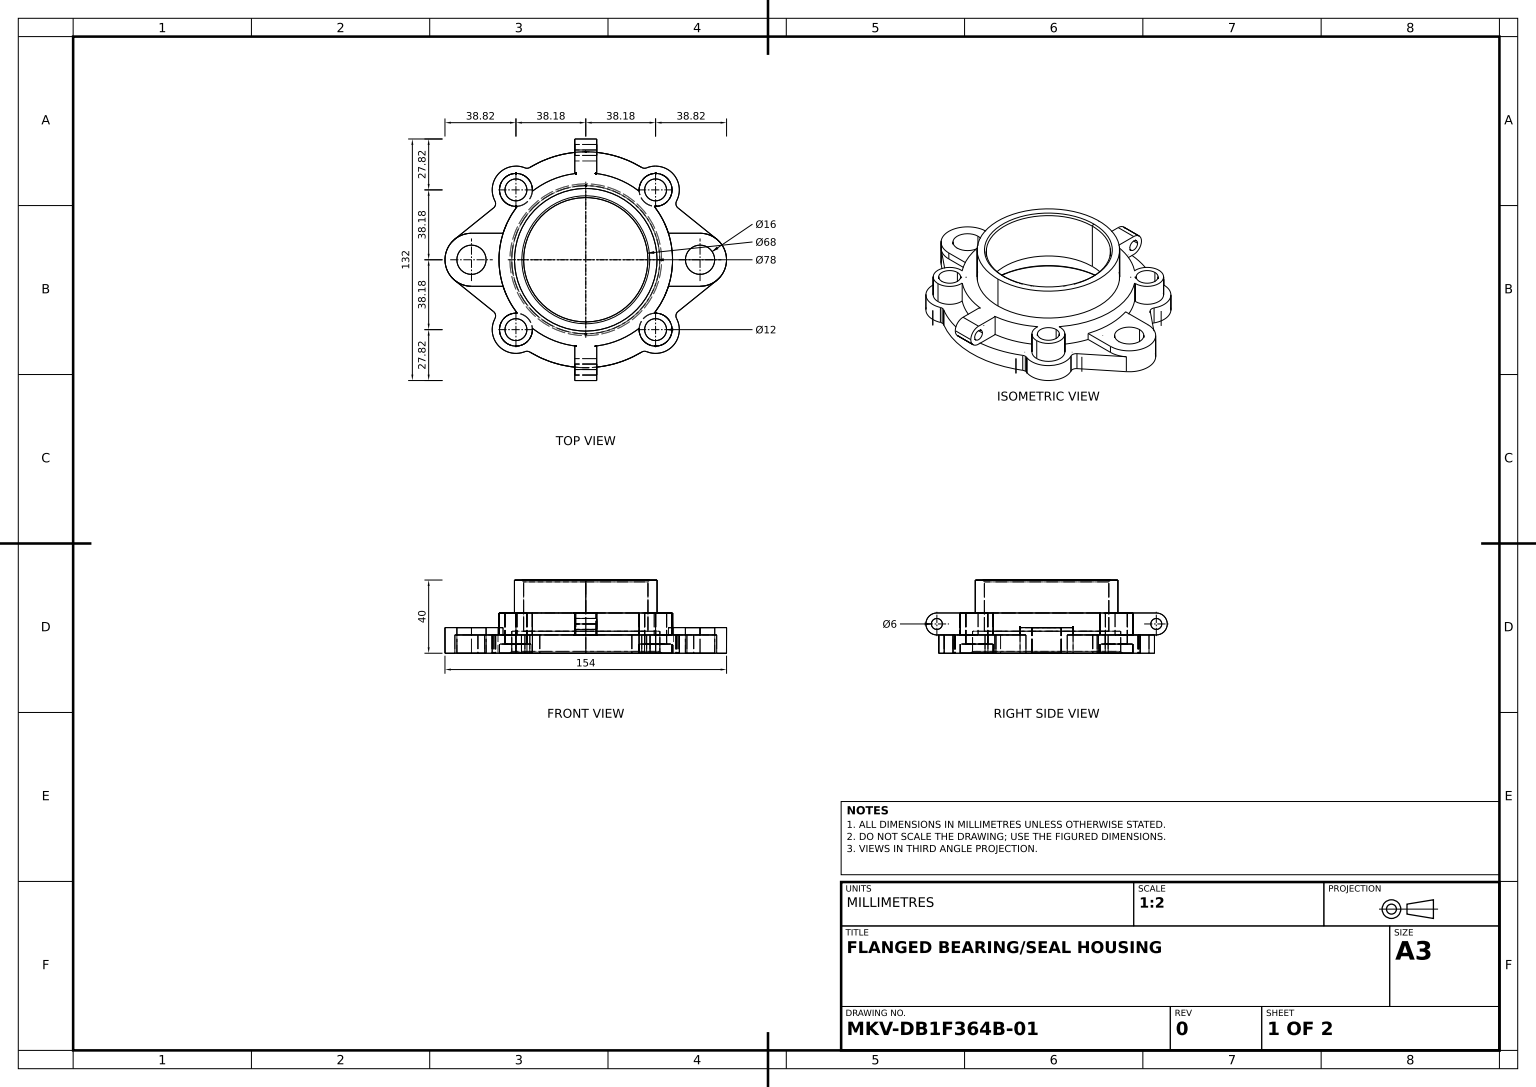
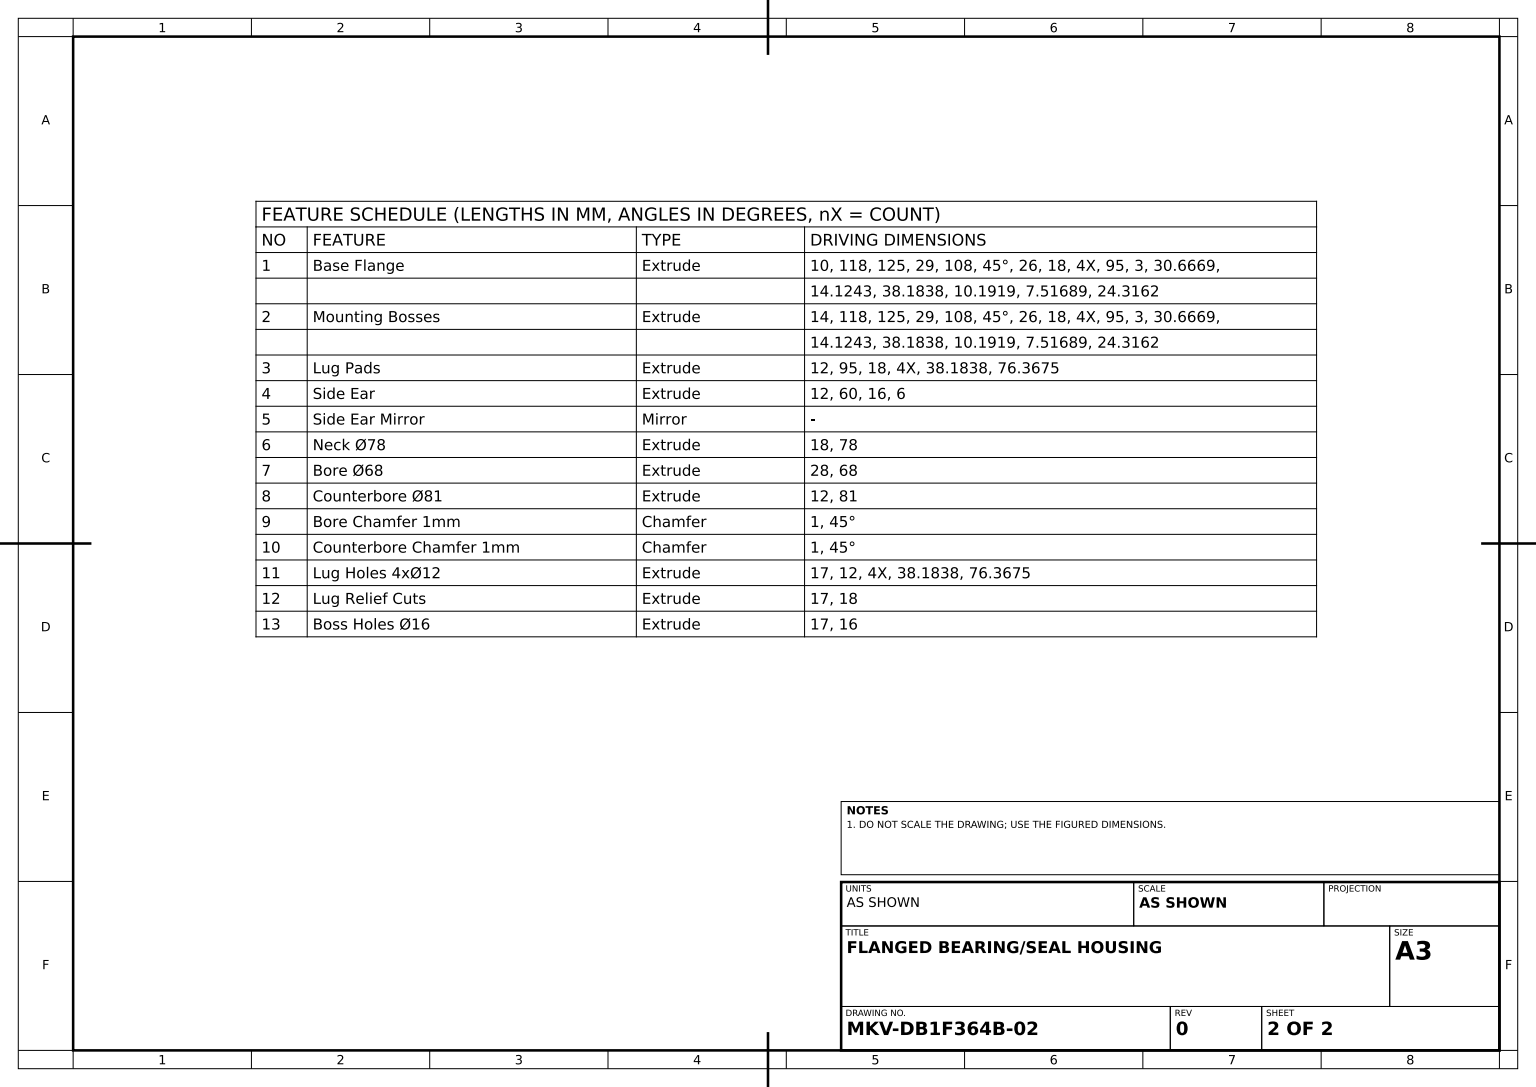
solid
v1 (38.183766,5,-32.183766)
v2 (38.183766,22,-32.183766)
e1 v1 v2 LINE
v3 (38.183766,22,-44.183766)
e2 v2 v3 CIRCLE(AX(P(38.183766,22,-38.183766),D(0,1,0),D(0,0,1)),6)
v4 (38.183766,5,-44.183766)
e3 v4 v3 LINE
e4 v1 v4 CIRCLE(AX(P(38.183766,5,-38.183766),D(0,1,0),D(0,0,1)),6)
face CYL(AX(P(38.183766,5,-38.183766),D(0,1,0),D(0,0,1)),6) rev [e1 e2 -e3 -e4]
v5 (6,16,-63)
v6 (-6,16,-63)
e5 v5 v6 LINE
v7 (6,16,-57)
e6 v7 v5 CIRCLE(AX(P(6,16,-60),D(-1,0,0),D(0,0,1)),3)
v8 (-6,16,-57)
e7 v7 v8 LINE
e8 v8 v6 CIRCLE(AX(P(-6,16,-60),D(-1,0,0),D(0,0,1)),3)
face CYL(AX(P(6,16,-60),D(-1,0,0),D(0,0,1)),3) rev [-e5 -e6 e7 e8]
v9 (-29.213373,22,37.454357)
v10 (-29.213373,10,37.454357)
e9 v9 v10 LINE
v11 (-38.183766,22,47.183766)
e10 v11 v9 CIRCLE(AX(P(-38.183766,22,38.183766),D(0,1,0),D(0,0,1)),9)
v12 (-38.183766,10,47.183766)
e11 v11 v12 LINE
e12 v12 v10 CIRCLE(AX(P(-38.183766,10,38.183766),D(0,1,0),D(0,0,1)),9)
face CYL(AX(P(-38.183766,22,38.183766),D(0,-1,0),D(0,0,-1)),9) [-e9 -e10 e11 e12]
v13 (-38.183766,0,-29.183766)
v14 (-38.183766,0,-47.183766)
e13 v13 v14 CIRCLE(AX(P(-38.183766,0,-38.183766),D(0,1,0),D(0,0,1)),9)
v15 (-38.183766,5,-29.183766)
e14 v13 v15 LINE
v16 (-38.183766,5,-47.183766)
e15 v15 v16 CIRCLE(AX(P(-38.183766,5,-38.183766),D(0,1,0),D(0,0,1)),9)
e16 v14 v16 LINE
face CYL(AX(P(-38.183766,-12,-38.183766),D(0,1,0),D(0,0,1)),9) rev [-e13 e14 e15 -e16]
v17 (38.183766,0,47.183766)
v18 (38.183766,5,47.183766)
e17 v17 v18 LINE
v19 (38.183766,5,29.183766)
e18 v18 v19 CIRCLE(AX(P(38.183766,5,38.183766),D(0,1,0),D(0,0,1)),9)
v20 (38.183766,0,29.183766)
e19 v20 v19 LINE
e20 v17 v20 CIRCLE(AX(P(38.183766,0,38.183766),D(0,1,0),D(0,0,1)),9)
face CYL(AX(P(38.183766,-12,38.183766),D(0,1,0),D(0,0,1)),9) rev [e17 e18 -e19 -e20]
v21 (38.183766,22,-47.183766)
v22 (38.183766,10,-47.183766)
e21 v21 v22 LINE
v23 (29.213373,10,-37.454357)
e22 v22 v23 CIRCLE(AX(P(38.183766,10,-38.183766),D(0,1,0),D(0,0,1)),9)
v24 (29.213373,22,-37.454357)
e23 v24 v23 LINE
e24 v21 v24 CIRCLE(AX(P(38.183766,22,-38.183766),D(0,1,0),D(0,0,1)),9)
face CYL(AX(P(38.183766,22,-38.183766),D(0,-1,0),D(0,0,-1)),9) [e21 e22 -e23 -e24]
v25 (-50.427104,0,-28.329799)
v26 (-71.591397,0,-11.295862)
e25 v25 v26 LINE
v27 (-71.591397,10,-11.295862)
e26 v27 v26 LINE
v28 (-50.427104,10,-28.329799)
e27 v28 v27 LINE
e28 v28 v25 LINE
face PLANE(AX(P(-33.661405,10,-41.823557),D(0.626992924,0,0.77902495),D(0.77902495,0,-0.626992924))) rev [e25 -e26 -e27 e28]
e29 v3 v2 CIRCLE(AX(P(38.183766,22,-38.183766),D(0,1,0),D(0,0,1)),6)
e30 v4 v1 CIRCLE(AX(P(38.183766,5,-38.183766),D(0,1,0),D(0,0,1)),6)
face CYL(AX(P(38.183766,5,-38.183766),D(0,1,0),D(0,0,1)),6) rev [e3 e29 -e1 -e30]
v29 (0,39,-34)
v30 (0,40,-35)
e31 v29 v30 LINE
v31 (0,39,34)
e32 v31 v29 CIRCLE(AX(P(0,39,0),D(0,1,0),D(0,0,1)),34)
v32 (0,40,35)
e33 v31 v32 LINE
e34 v30 v32 CIRCLE(AX(P(0,40,0),D(0,-1,0),D(0,0,1)),35)
face CONE(AX(P(0,39,0),D(0,1,0),D(0,0,1)),34,0.785398163) rev [-e31 -e32 e33 -e34]
v33 (62.5,0,-8)
v34 (62.5,14,-8)
e35 v33 v34 LINE
v35 (62.5,14,8)
e36 v34 v35 CIRCLE(AX(P(62.5,14,0),D(0,1,0),D(0,0,1)),8)
v36 (62.5,0,8)
e37 v36 v35 LINE
e38 v33 v36 CIRCLE(AX(P(62.5,0,0),D(0,1,0),D(0,0,1)),8)
face CYL(AX(P(62.5,-3,0),D(0,1,0),D(0,0,1)),8) rev [e35 e36 -e37 -e38]
v37 (0,10,-59)
v38 (0,0,-59)
e39 v37 v38 LINE
v39 (6,10,-58.694122)
e40 v37 v39 CIRCLE(AX(P(0,10,0),D(0,-1,0),D(0,0,-1)),59)
v40 (30.604247,10,-50.441848)
e41 v40 v39 CIRCLE(AX(P(0,10,0),D(0,1,0),D(0,0,1)),59)
v41 (30.604247,0,-50.441848)
e42 v40 v41 LINE
e43 v41 v38 CIRCLE(AX(P(0,0,0),D(0,1,0),D(0,0,1)),59)
face CYL(AX(P(0,10,0),D(0,-1,0),D(0,0,-1)),59) [-e39 e40 -e41 e42 e43]
v42 (29.213373,22,37.454357)
v43 (29.213373,10,37.454357)
e44 v42 v43 LINE
v44 (38.183766,10,47.183766)
e45 v43 v44 CIRCLE(AX(P(38.183766,10,38.183766),D(0,1,0),D(0,0,1)),9)
v45 (38.183766,22,47.183766)
e46 v45 v44 LINE
e47 v42 v45 CIRCLE(AX(P(38.183766,22,38.183766),D(0,1,0),D(0,0,1)),9)
face CYL(AX(P(38.183766,22,38.183766),D(0,-1,0),D(0,0,-1)),9) [e44 e45 -e46 -e47]
v46 (-37.454357,22,29.213373)
v47 (-37.454357,10,29.213373)
e48 v46 v47 LINE
v48 (-38.183766,10,29.183766)
e49 v47 v48 CIRCLE(AX(P(-38.183766,10,38.183766),D(0,1,0),D(0,0,1)),9)
v49 (-38.183766,22,29.183766)
e50 v49 v48 LINE
e51 v46 v49 CIRCLE(AX(P(-38.183766,22,38.183766),D(0,1,0),D(0,0,1)),9)
face CYL(AX(P(-38.183766,22,38.183766),D(0,-1,0),D(0,0,-1)),9) [e48 e49 -e50 -e51]
v50 (-38.183766,5,29.183766)
v51 (-38.183766,5,47.183766)
e52 v50 v51 CIRCLE(AX(P(-38.183766,5,38.183766),D(0,1,0),D(0,0,1)),9)
v52 (-38.183766,0,47.183766)
e53 v52 v51 LINE
v53 (-38.183766,0,29.183766)
e54 v53 v52 CIRCLE(AX(P(-38.183766,0,38.183766),D(0,1,0),D(0,0,1)),9)
e55 v53 v50 LINE
face CYL(AX(P(-38.183766,-12,38.183766),D(0,1,0),D(0,0,1)),9) rev [e52 -e53 -e54 e55]
v54 (0,40,39)
v55 (0,40,-39)
e56 v54 v55 CIRCLE(AX(P(0,40,0),D(0,1,0),D(0,0,1)),39)
v56 (0,22,39)
e57 v54 v56 LINE
v57 (0,22,-39)
e58 v56 v57 CIRCLE(AX(P(0,22,0),D(0,1,0),D(0,0,1)),39)
e59 v55 v57 LINE
face CYL(AX(P(0,40,0),D(0,-1,0),D(0,0,-1)),39) [-e56 e57 e58 -e59]
v58 (38.183766,0,-29.183766)
v59 (38.183766,5,-29.183766)
e60 v58 v59 LINE
v60 (38.183766,5,-47.183766)
e61 v59 v60 CIRCLE(AX(P(38.183766,5,-38.183766),D(0,1,0),D(0,0,1)),9)
v61 (38.183766,0,-47.183766)
e62 v61 v60 LINE
e63 v58 v61 CIRCLE(AX(P(38.183766,0,-38.183766),D(0,1,0),D(0,0,1)),9)
face CYL(AX(P(38.183766,-12,-38.183766),D(0,1,0),D(0,0,1)),9) rev [e60 e61 -e62 -e63]
e64 v5 v7 CIRCLE(AX(P(6,16,-60),D(-1,0,0),D(0,0,1)),3)
e65 v6 v8 CIRCLE(AX(P(-6,16,-60),D(-1,0,0),D(0,0,1)),3)
face CYL(AX(P(6,16,-60),D(-1,0,0),D(0,0,1)),3) rev [-e64 e5 e65 -e7]
v62 (38.183766,22,-29.183766)
e66 v62 v21 CIRCLE(AX(P(38.183766,22,-38.183766),D(0,1,0),D(0,0,1)),9)
v63 (38.183766,10,-29.183766)
e67 v62 v63 LINE
e68 v63 v22 CIRCLE(AX(P(38.183766,10,-38.183766),D(0,1,0),D(0,0,1)),9)
face CYL(AX(P(38.183766,22,-38.183766),D(0,-1,0),D(0,0,-1)),9) [-e66 e67 e68 -e21]
v64 (38.183766,5,44.183766)
v65 (38.183766,5,32.183766)
e69 v64 v65 CIRCLE(AX(P(38.183766,5,38.183766),D(0,1,0),D(0,0,1)),6)
v66 (38.183766,22,44.183766)
e70 v64 v66 LINE
v67 (38.183766,22,32.183766)
e71 v66 v67 CIRCLE(AX(P(38.183766,22,38.183766),D(0,1,0),D(0,0,1)),6)
e72 v65 v67 LINE
face CYL(AX(P(38.183766,5,38.183766),D(0,1,0),D(0,0,1)),6) rev [-e69 e70 e71 -e72]
v68 (-38.183766,5,44.183766)
v69 (-38.183766,5,32.183766)
e73 v68 v69 CIRCLE(AX(P(-38.183766,5,38.183766),D(0,1,0),D(0,0,1)),6)
e74 v69 v68 CIRCLE(AX(P(-38.183766,5,38.183766),D(0,1,0),D(0,0,1)),6)
e75 v51 v50 CIRCLE(AX(P(-38.183766,5,38.183766),D(0,1,0),D(0,0,1)),9)
face PLANE(AX(P(-38.183766,5,38.183766),D(0,1,0),D(0,0,1))) rev [e73 e74] [-e75 -e52]
v70 (-62.5,0,8)
v71 (-62.5,0,-8)
e76 v70 v71 CIRCLE(AX(P(-62.5,0,0),D(0,1,0),D(0,0,1)),8)
v72 (-62.5,14,8)
e77 v70 v72 LINE
v73 (-62.5,14,-8)
e78 v72 v73 CIRCLE(AX(P(-62.5,14,0),D(0,1,0),D(0,0,1)),8)
e79 v71 v73 LINE
face CYL(AX(P(-62.5,-3,0),D(0,1,0),D(0,0,1)),8) rev [-e76 e77 e78 -e79]
v74 (-62.5,14,-14.5)
v75 (-45.232732,14,-14.5)
e80 v74 v75 LINE
v76 (-45.232732,10,-14.5)
e81 v75 v76 LINE
v77 (-62.5,10,-14.5)
e82 v77 v76 LINE
e83 v74 v77 LINE
face PLANE(AX(P(0,14,-14.5),D(0,0,-1),D(-1,0,0))) [e80 e81 -e82 -e83]
e84 v55 v54 CIRCLE(AX(P(0,40,0),D(0,1,0),D(0,0,1)),39)
e85 v32 v30 CIRCLE(AX(P(0,40,0),D(0,-1,0),D(0,0,1)),35)
face PLANE(AX(P(0,40,0),D(0,1,0),D(0,0,1))) [e84 e56] [e85 e34]
v78 (37.454357,10,-29.213373)
e86 v78 v63 CIRCLE(AX(P(38.183766,10,-38.183766),D(0,1,0),D(0,0,1)),9)
v79 (37.454357,22,-29.213373)
e87 v79 v62 CIRCLE(AX(P(38.183766,22,-38.183766),D(0,1,0),D(0,0,1)),9)
e88 v79 v78 LINE
face CYL(AX(P(38.183766,22,-38.183766),D(0,-1,0),D(0,0,-1)),9) [e86 -e67 -e87 e88]
v80 (-49.659774,10,-32.076291)
e89 v28 v80 CIRCLE(AX(P(-52.308083,10,-30.666874),D(0,1,0),D(0,0,1)),3)
v81 (-49.659774,0,-32.076291)
e90 v80 v81 LINE
e91 v25 v81 CIRCLE(AX(P(-52.308083,0,-30.666874),D(0,1,0),D(0,0,1)),3)
face CYL(AX(P(-52.308083,10,-30.666874),D(0,-1,0),D(0,0,-1)),3) rev [-e28 e89 e90 -e91]
e92 v35 v34 CIRCLE(AX(P(62.5,14,0),D(0,1,0),D(0,0,1)),8)
v82 (62.5,14,14.5)
v83 (62.5,14,-14.5)
e93 v82 v83 CIRCLE(AX(P(62.5,14,0),D(0,1,0),D(0,0,1)),14.5)
v84 (45.232732,14,-14.5)
e94 v83 v84 LINE
v85 (45.232732,14,14.5)
e95 v85 v84 CIRCLE(AX(P(0,14,0),D(0,1,0),D(0,0,1)),47.5)
e96 v82 v85 LINE
face PLANE(AX(P(0,14,0),D(0,1,0),D(0,0,1))) [-e92 -e36] [e93 e94 -e95 -e96]
v86 (0,12,34)
e97 v86 v31 LINE
v87 (0,12,-34)
e98 v87 v29 LINE
e99 v86 v87 CIRCLE(AX(P(0,12,0),D(0,1,0),D(0,0,1)),34)
face CYL(AX(P(0,12,0),D(0,1,0),D(0,0,1)),34) rev [e97 e32 -e98 -e99]
v88 (5.471947,10,47.183766)
v89 (5.471947,22,47.183766)
e100 v88 v89 LINE
e101 v88 v43 CIRCLE(AX(P(0,10,0),D(0,1,0),D(0,0,1)),47.5)
e102 v89 v42 CIRCLE(AX(P(0,22,0),D(0,1,0),D(0,0,1)),47.5)
face CYL(AX(P(0,22,0),D(0,-1,0),D(0,0,-1)),47.5) [-e100 e101 -e44 -e102]
v90 (6,16,57)
v91 (-6,16,57)
e103 v90 v91 LINE
v92 (6,16,63)
e104 v90 v92 CIRCLE(AX(P(6,16,60),D(1,0,0),D(0,0,-1)),3)
v93 (-6,16,63)
e105 v92 v93 LINE
e106 v91 v93 CIRCLE(AX(P(-6,16,60),D(1,0,0),D(0,0,-1)),3)
face CYL(AX(P(6,16,60),D(-1,0,0),D(0,0,1)),3) rev [-e103 e104 e105 -e106]
v94 (-6,10,-58.694122)
e107 v94 v37 CIRCLE(AX(P(0,10,0),D(0,-1,0),D(0,0,-1)),59)
v95 (-30.604247,0,-50.441848)
e108 v38 v95 CIRCLE(AX(P(0,0,0),D(0,1,0),D(0,0,1)),59)
v96 (-30.604247,10,-50.441848)
e109 v96 v95 LINE
e110 v94 v96 CIRCLE(AX(P(0,10,0),D(0,1,0),D(0,0,1)),59)
face CYL(AX(P(0,10,0),D(0,-1,0),D(0,0,-1)),59) [e107 e39 e108 -e109 -e110]
v97 (62.5,10,14.5)
v98 (45.232732,10,14.5)
e111 v97 v98 LINE
e112 v82 v97 LINE
e113 v85 v98 LINE
face PLANE(AX(P(0,14,14.5),D(0,0,1),D(1,0,0))) [-e111 -e112 e96 e113]
e114 v16 v15 CIRCLE(AX(P(-38.183766,5,-38.183766),D(0,1,0),D(0,0,1)),9)
e115 v14 v13 CIRCLE(AX(P(-38.183766,0,-38.183766),D(0,1,0),D(0,0,1)),9)
face CYL(AX(P(-38.183766,-12,-38.183766),D(0,1,0),D(0,0,1)),9) rev [e114 -e14 -e115 e16]
v99 (32.160396,10,50.006688)
v100 (32.160396,0,50.006688)
e116 v99 v100 LINE
v101 (30.604247,10,50.441848)
e117 v99 v101 CIRCLE(AX(P(32.160396,10,53.006688),D(0,1,0),D(0,0,1)),3)
v102 (30.604247,0,50.441848)
e118 v101 v102 LINE
e119 v100 v102 CIRCLE(AX(P(32.160396,0,53.006688),D(0,1,0),D(0,0,1)),3)
face CYL(AX(P(32.160396,10,53.006688),D(0,-1,0),D(0,0,-1)),3) rev [-e116 e117 e118 -e119]
v103 (45.232732,10,-14.5)
e120 v103 v78 CIRCLE(AX(P(0,10,0),D(0,1,0),D(0,0,1)),47.5)
v104 (37.454357,22,29.213373)
e121 v104 v79 CIRCLE(AX(P(0,22,0),D(0,1,0),D(0,0,1)),47.5)
v105 (37.454357,10,29.213373)
e122 v104 v105 LINE
e123 v105 v98 CIRCLE(AX(P(0,10,0),D(0,1,0),D(0,0,1)),47.5)
e124 v84 v103 LINE
face CYL(AX(P(0,22,0),D(0,-1,0),D(0,0,-1)),47.5) [e120 -e88 -e121 e122 e123 -e113 e95 e124]
v106 (-38.183766,22,-29.183766)
v107 (-38.183766,10,-29.183766)
e125 v106 v107 LINE
v108 (-37.454357,10,-29.213373)
e126 v107 v108 CIRCLE(AX(P(-38.183766,10,-38.183766),D(0,1,0),D(0,0,1)),9)
v109 (-37.454357,22,-29.213373)
e127 v109 v108 LINE
e128 v106 v109 CIRCLE(AX(P(-38.183766,22,-38.183766),D(0,1,0),D(0,0,1)),9)
face CYL(AX(P(-38.183766,22,-38.183766),D(0,-1,0),D(0,0,-1)),9) [e125 e126 -e127 -e128]
v110 (-5.471947,22,47.183766)
v111 (-5.471947,10,47.183766)
e129 v110 v111 LINE
v112 (-6,10,47.183766)
e130 v111 v112 LINE
v113 (-6,22,47.183766)
e131 v112 v113 LINE
e132 v110 v113 LINE
face PLANE(AX(P(6,10,47.183766),D(0,0,1),D(1,0,0))) rev [e129 e130 e131 -e132]
v114 (6,10,60)
v115 (-6,10,60)
e133 v114 v115 LINE
v116 (6,16,66)
e134 v116 v114 CIRCLE(AX(P(6,16,60),D(1,0,0),D(0,0,-1)),6)
v117 (-6,16,66)
e135 v116 v117 LINE
e136 v117 v115 CIRCLE(AX(P(-6,16,60),D(1,0,0),D(0,0,-1)),6)
face CYL(AX(P(6,16,60),D(-1,0,0),D(0,0,1)),6) [-e133 -e134 e135 e136]
v118 (5.471947,22,-47.183766)
e137 v24 v118 CIRCLE(AX(P(0,22,0),D(0,1,0),D(0,0,1)),47.5)
v119 (5.471947,10,-47.183766)
e138 v23 v119 CIRCLE(AX(P(0,10,0),D(0,1,0),D(0,0,1)),47.5)
e139 v119 v118 LINE
face CYL(AX(P(0,22,0),D(0,-1,0),D(0,0,-1)),47.5) [-e137 e23 e138 e139]
v120 (-49.659774,10,32.076291)
v121 (-33.289778,10,50.22739)
e140 v120 v121 CIRCLE(AX(P(-38.183766,10,38.183766),D(0,1,0),D(0,0,1)),13)
v122 (-32.160396,10,50.006688)
e141 v122 v121 CIRCLE(AX(P(-32.160396,10,53.006688),D(0,1,0),D(0,0,1)),3)
v123 (-30.604247,10,50.441848)
e142 v123 v122 CIRCLE(AX(P(-32.160396,10,53.006688),D(0,1,0),D(0,0,1)),3)
v124 (-6,10,58.694122)
e143 v123 v124 CIRCLE(AX(P(0,10,0),D(0,1,0),D(0,0,1)),59)
e144 v124 v112 LINE
e145 v10 v111 CIRCLE(AX(P(0,10,0),D(0,1,0),D(0,0,1)),47.5)
e146 v48 v12 CIRCLE(AX(P(-38.183766,10,38.183766),D(0,1,0),D(0,0,1)),9)
v125 (-45.232732,10,14.5)
e147 v125 v47 CIRCLE(AX(P(0,10,0),D(0,1,0),D(0,0,1)),47.5)
v126 (-62.5,10,14.5)
e148 v126 v125 LINE
v127 (-71.591397,10,11.295862)
e149 v127 v126 CIRCLE(AX(P(-62.5,10,0),D(0,1,0),D(0,0,1)),14.5)
v128 (-50.427104,10,28.329799)
e150 v128 v127 LINE
e151 v120 v128 CIRCLE(AX(P(-52.308083,10,30.666874),D(0,1,0),D(0,0,1)),3)
face PLANE(AX(P(0,10,0),D(0,1,0),D(0,0,1))) [e140 -e141 -e142 e143 e144 -e130 -e145 -e12 -e146 -e49 -e147 -e148 -e149 -e150 -e151]
v129 (-33.289778,0,50.22739)
e152 v121 v129 LINE
v130 (-32.160396,0,50.006688)
e153 v130 v129 CIRCLE(AX(P(-32.160396,0,53.006688),D(0,1,0),D(0,0,1)),3)
e154 v122 v130 LINE
face CYL(AX(P(-32.160396,10,53.006688),D(0,-1,0),D(0,0,-1)),3) rev [e141 e152 -e153 -e154]
e155 v108 v76 CIRCLE(AX(P(0,10,0),D(0,1,0),D(0,0,1)),47.5)
v131 (-38.183766,10,-47.183766)
e156 v131 v107 CIRCLE(AX(P(-38.183766,10,-38.183766),D(0,1,0),D(0,0,1)),9)
v132 (-29.213373,10,-37.454357)
e157 v132 v131 CIRCLE(AX(P(-38.183766,10,-38.183766),D(0,1,0),D(0,0,1)),9)
v133 (-5.471947,10,-47.183766)
e158 v133 v132 CIRCLE(AX(P(0,10,0),D(0,1,0),D(0,0,1)),47.5)
v134 (-6,10,-47.183766)
e159 v133 v134 LINE
e160 v94 v134 LINE
v135 (-33.289778,10,-50.22739)
e161 v96 v135 CIRCLE(AX(P(-32.160396,10,-53.006688),D(0,-1,0),D(0,0,1)),3)
v136 (-38.183766,10,-51.183766)
e162 v135 v136 CIRCLE(AX(P(-38.183766,10,-38.183766),D(0,1,0),D(0,0,1)),13)
e163 v136 v80 CIRCLE(AX(P(-38.183766,10,-38.183766),D(0,1,0),D(0,0,1)),13)
e164 v77 v27 CIRCLE(AX(P(-62.5,10,0),D(0,1,0),D(0,0,1)),14.5)
face PLANE(AX(P(0,10,0),D(0,1,0),D(0,0,1))) [e82 -e155 -e126 -e156 -e157 -e158 e159 -e160 e110 e161 e162 e163 -e89 e27 -e164]
v137 (-38.183766,22,-47.183766)
e165 v137 v106 CIRCLE(AX(P(-38.183766,22,-38.183766),D(0,1,0),D(0,0,1)),9)
e166 v137 v131 LINE
face CYL(AX(P(-38.183766,22,-38.183766),D(0,-1,0),D(0,0,-1)),9) [-e125 -e165 e166 e156]
v138 (-38.183766,22,44.183766)
e167 v68 v138 LINE
v139 (-38.183766,22,32.183766)
e168 v138 v139 CIRCLE(AX(P(-38.183766,22,38.183766),D(0,1,0),D(0,0,1)),6)
e169 v69 v139 LINE
face CYL(AX(P(-38.183766,5,38.183766),D(0,1,0),D(0,0,1)),6) rev [-e73 e167 e168 -e169]
v140 (49.659774,10,-32.076291)
v141 (49.659774,0,-32.076291)
e170 v140 v141 LINE
v142 (50.427104,10,-28.329799)
e171 v142 v140 CIRCLE(AX(P(52.308083,10,-30.666874),D(0,-1,0),D(0,0,1)),3)
v143 (50.427104,0,-28.329799)
e172 v142 v143 LINE
e173 v143 v141 CIRCLE(AX(P(52.308083,0,-30.666874),D(0,-1,0),D(0,0,1)),3)
face CYL(AX(P(52.308083,10,-30.666874),D(0,-1,0),D(0,0,-1)),3) rev [-e170 -e171 e172 e173]
v144 (6,22,60)
e174 v144 v116 CIRCLE(AX(P(6,16,60),D(1,0,0),D(0,0,-1)),6)
v145 (-6,22,60)
e175 v144 v145 LINE
e176 v145 v117 CIRCLE(AX(P(-6,16,60),D(1,0,0),D(0,0,-1)),6)
face CYL(AX(P(6,16,60),D(-1,0,0),D(0,0,1)),6) [-e135 -e174 e175 e176]
v146 (71.591397,0,-11.295862)
e177 v143 v146 LINE
v147 (71.591397,10,-11.295862)
e178 v142 v147 LINE
e179 v147 v146 LINE
face PLANE(AX(P(33.661405,10,-41.823557),D(0.626992924,0,-0.77902495),D(-0.77902495,0,-0.626992924))) [-e177 -e172 e178 e179]
e180 v19 v18 CIRCLE(AX(P(38.183766,5,38.183766),D(0,1,0),D(0,0,1)),9)
e181 v20 v17 CIRCLE(AX(P(38.183766,0,38.183766),D(0,1,0),D(0,0,1)),9)
face CYL(AX(P(38.183766,-12,38.183766),D(0,1,0),D(0,0,1)),9) rev [e19 e180 -e17 -e181]
v148 (-29.213373,22,-37.454357)
e182 v148 v137 CIRCLE(AX(P(-38.183766,22,-38.183766),D(0,1,0),D(0,0,1)),9)
e183 v148 v132 LINE
face CYL(AX(P(-38.183766,22,-38.183766),D(0,-1,0),D(0,0,-1)),9) [-e182 e183 e157 -e166]
v149 (-30.604247,0,50.441848)
e184 v149 v130 CIRCLE(AX(P(-32.160396,0,53.006688),D(0,1,0),D(0,0,1)),3)
e185 v123 v149 LINE
face CYL(AX(P(-32.160396,10,53.006688),D(0,-1,0),D(0,0,-1)),3) rev [-e184 -e185 e142 e154]
v150 (-33.289778,0,-50.22739)
e186 v95 v150 CIRCLE(AX(P(-32.160396,0,-53.006688),D(0,-1,0),D(0,0,1)),3)
e187 v135 v150 LINE
face CYL(AX(P(-32.160396,10,-53.006688),D(0,-1,0),D(0,0,-1)),3) rev [e186 -e187 -e161 e109]
v151 (-38.183766,5,-32.183766)
v152 (-38.183766,5,-44.183766)
e188 v151 v152 CIRCLE(AX(P(-38.183766,5,-38.183766),D(0,1,0),D(0,0,1)),6)
e189 v152 v151 CIRCLE(AX(P(-38.183766,5,-38.183766),D(0,1,0),D(0,0,1)),6)
face PLANE(AX(P(-38.183766,5,-38.183766),D(0,1,0),D(0,0,1))) rev [e188 e189] [-e114 -e15]
v153 (62.5,10,-14.5)
e190 v83 v153 LINE
e191 v153 v103 LINE
face PLANE(AX(P(0,14,-14.5),D(0,0,1),D(1,0,0))) rev [e190 e191 -e124 -e94]
v154 (71.591397,0,11.295862)
e192 v154 v146 CIRCLE(AX(P(62.5,0,0),D(0,1,0),D(0,0,1)),14.5)
v155 (50.427104,0,28.329799)
e193 v155 v154 LINE
v156 (49.659774,0,32.076291)
e194 v156 v155 CIRCLE(AX(P(52.308083,0,30.666874),D(0,-1,0),D(0,0,1)),3)
v157 (33.289778,0,50.22739)
e195 v157 v156 CIRCLE(AX(P(38.183766,0,38.183766),D(0,1,0),D(0,0,1)),13)
e196 v157 v100 CIRCLE(AX(P(32.160396,0,53.006688),D(0,1,0),D(0,0,1)),3)
e197 v149 v102 CIRCLE(AX(P(0,0,0),D(0,1,0),D(0,0,1)),59)
v158 (-49.659774,0,32.076291)
e198 v158 v129 CIRCLE(AX(P(-38.183766,0,38.183766),D(0,1,0),D(0,0,1)),13)
v159 (-50.427104,0,28.329799)
e199 v158 v159 CIRCLE(AX(P(-52.308083,0,30.666874),D(0,1,0),D(0,0,1)),3)
v160 (-71.591397,0,11.295862)
e200 v159 v160 LINE
e201 v26 v160 CIRCLE(AX(P(-62.5,0,0),D(0,1,0),D(0,0,1)),14.5)
v161 (-38.183766,0,-51.183766)
e202 v161 v81 CIRCLE(AX(P(-38.183766,0,-38.183766),D(0,1,0),D(0,0,1)),13)
e203 v150 v161 CIRCLE(AX(P(-38.183766,0,-38.183766),D(0,1,0),D(0,0,1)),13)
v162 (33.289778,0,-50.22739)
e204 v162 v41 CIRCLE(AX(P(32.160396,0,-53.006688),D(0,-1,0),D(0,0,1)),3)
v163 (38.183766,0,-51.183766)
e205 v163 v162 CIRCLE(AX(P(38.183766,0,-38.183766),D(0,1,0),D(0,0,1)),13)
e206 v141 v163 CIRCLE(AX(P(38.183766,0,-38.183766),D(0,1,0),D(0,0,1)),13)
v164 (0,0,-41.5)
v165 (0,0,41.5)
e207 v164 v165 CIRCLE(AX(P(0,0,0),D(0,1,0),D(0,0,1)),41.5)
e208 v165 v164 CIRCLE(AX(P(0,0,0),D(0,1,0),D(0,0,1)),41.5)
e209 v71 v70 CIRCLE(AX(P(-62.5,0,0),D(0,1,0),D(0,0,1)),8)
e210 v61 v58 CIRCLE(AX(P(38.183766,0,-38.183766),D(0,1,0),D(0,0,1)),9)
e211 v36 v33 CIRCLE(AX(P(62.5,0,0),D(0,1,0),D(0,0,1)),8)
e212 v52 v53 CIRCLE(AX(P(-38.183766,0,38.183766),D(0,1,0),D(0,0,1)),9)
face PLANE(AX(P(0,0,0),D(0,1,0),D(0,0,1))) rev [e115 e13] [-e192 -e193 -e194 -e195 e196 e119 -e197 e184 e153 -e198 e199 e200 -e201 -e25 e91 -e202 -e203 -e186 -e108 -e43 -e204 -e205 -e206 -e173 e177] [e207 e208] [e209 e76] [e181 e20] [e210 e63] [e211 e38] [e54 e212]
e213 v87 v86 CIRCLE(AX(P(0,12,0),D(0,1,0),D(0,0,1)),34)
v166 (0,12,40.5)
v167 (0,12,-40.5)
e214 v166 v167 CIRCLE(AX(P(0,12,0),D(0,1,0),D(0,0,1)),40.5)
e215 v167 v166 CIRCLE(AX(P(0,12,0),D(0,1,0),D(0,0,1)),40.5)
face PLANE(AX(P(0,12,0),D(0,1,0),D(0,0,1))) rev [e213 e99] [-e214 -e215]
e216 v29 v31 CIRCLE(AX(P(0,39,0),D(0,1,0),D(0,0,1)),34)
face CYL(AX(P(0,12,0),D(0,1,0),D(0,0,1)),34) rev [-e213 e98 e216 -e97]
e217 v9 v110 CIRCLE(AX(P(0,22,0),D(0,1,0),D(0,0,1)),47.5)
face CYL(AX(P(0,22,0),D(0,-1,0),D(0,0,-1)),47.5) [-e217 e9 e145 -e129]
e218 v139 v138 CIRCLE(AX(P(-38.183766,22,38.183766),D(0,1,0),D(0,0,1)),6)
e219 v49 v11 CIRCLE(AX(P(-38.183766,22,38.183766),D(0,1,0),D(0,0,1)),9)
e220 v113 v145 LINE
v168 (6,22,47.183766)
e221 v168 v144 LINE
e222 v168 v89 LINE
v169 (38.183766,22,29.183766)
e223 v45 v169 CIRCLE(AX(P(38.183766,22,38.183766),D(0,1,0),D(0,0,1)),9)
e224 v169 v104 CIRCLE(AX(P(38.183766,22,38.183766),D(0,1,0),D(0,0,1)),9)
v170 (6,22,-47.183766)
e225 v170 v118 LINE
v171 (6,22,-60)
e226 v170 v171 LINE
v172 (-6,22,-60)
e227 v171 v172 LINE
v173 (-6,22,-47.183766)
e228 v173 v172 LINE
v174 (-5.471947,22,-47.183766)
e229 v174 v173 LINE
e230 v174 v148 CIRCLE(AX(P(0,22,0),D(0,1,0),D(0,0,1)),47.5)
e231 v109 v46 CIRCLE(AX(P(0,22,0),D(0,1,0),D(0,0,1)),47.5)
v175 (-38.183766,22,-32.183766)
v176 (-38.183766,22,-44.183766)
e232 v175 v176 CIRCLE(AX(P(-38.183766,22,-38.183766),D(0,1,0),D(0,0,1)),6)
e233 v176 v175 CIRCLE(AX(P(-38.183766,22,-38.183766),D(0,1,0),D(0,0,1)),6)
e234 v67 v66 CIRCLE(AX(P(38.183766,22,38.183766),D(0,1,0),D(0,0,1)),6)
e235 v57 v56 CIRCLE(AX(P(0,22,0),D(0,1,0),D(0,0,1)),39)
face PLANE(AX(P(0,22,0),D(0,1,0),D(0,0,1))) [-e218 -e168] [e51 e219 e10 e217 e132 e220 -e175 -e221 e222 e102 e47 e223 e224 e121 e87 e66 e24 e137 -e225 e226 e227 -e228 -e229 e230 e182 e165 e128 e231] [-e232 -e233] [-e29 -e2] [-e71 -e234] [-e235 -e58]
v177 (38.183766,10,29.183766)
e236 v44 v177 CIRCLE(AX(P(38.183766,10,38.183766),D(0,1,0),D(0,0,1)),9)
e237 v169 v177 LINE
face CYL(AX(P(38.183766,22,38.183766),D(0,-1,0),D(0,0,-1)),9) [e236 -e237 -e223 e46]
e238 v134 v173 LINE
e239 v174 v133 LINE
face PLANE(AX(P(6,10,-47.183766),D(0,0,1),D(1,0,0))) [e229 -e238 -e159 -e239]
v178 (6,10,58.694122)
e240 v114 v178 LINE
e241 v115 v124 LINE
e242 v124 v178 CIRCLE(AX(P(0,10,0),D(0,1,0),D(0,0,1)),59)
face PLANE(AX(P(6,10,60),D(0,1,0),D(0,0,1))) rev [-e240 e133 e241 e242]
v179 (-45.232732,14,14.5)
e243 v75 v179 CIRCLE(AX(P(0,14,0),D(0,1,0),D(0,0,1)),47.5)
e244 v179 v125 LINE
face CYL(AX(P(0,22,0),D(0,-1,0),D(0,0,-1)),47.5) [-e81 e243 e244 e147 -e48 -e231 e127 e155]
face CYL(AX(P(-38.183766,-12,38.183766),D(0,1,0),D(0,0,1)),9) rev [-e55 -e212 e53 e75]
e245 v177 v105 CIRCLE(AX(P(38.183766,10,38.183766),D(0,1,0),D(0,0,1)),9)
face CYL(AX(P(38.183766,22,38.183766),D(0,-1,0),D(0,0,-1)),9) [-e224 e237 e245 -e122]
e246 v65 v64 CIRCLE(AX(P(38.183766,5,38.183766),D(0,1,0),D(0,0,1)),6)
face PLANE(AX(P(38.183766,5,38.183766),D(0,1,0),D(0,0,1))) rev [e69 e246] [-e180 -e18]
v180 (38.183766,10,-51.183766)
e247 v180 v163 LINE
e248 v140 v180 CIRCLE(AX(P(38.183766,10,-38.183766),D(0,1,0),D(0,0,1)),13)
face CYL(AX(P(38.183766,10,-38.183766),D(0,-1,0),D(0,0,-1)),13) [e170 e206 -e247 -e248]
face CYL(AX(P(-38.183766,22,38.183766),D(0,-1,0),D(0,0,-1)),9) [e146 -e11 -e219 e50]
face CYL(AX(P(38.183766,5,38.183766),D(0,1,0),D(0,0,1)),6) rev [e72 e234 -e70 -e246]
v181 (6,10,-47.183766)
e249 v181 v119 LINE
e250 v181 v170 LINE
face PLANE(AX(P(6,10,-47.183766),D(0,0,1),D(1,0,0))) [-e139 -e249 e250 e225]
e251 v60 v59 CIRCLE(AX(P(38.183766,5,-38.183766),D(0,1,0),D(0,0,1)),9)
face CYL(AX(P(38.183766,-12,-38.183766),D(0,1,0),D(0,0,1)),9) rev [-e210 e62 e251 -e60]
e252 v136 v161 LINE
face CYL(AX(P(-38.183766,10,-38.183766),D(0,-1,0),D(0,0,-1)),13) [e202 -e90 -e163 e252]
e253 v178 v101 CIRCLE(AX(P(0,10,0),D(0,1,0),D(0,0,1)),59)
face CYL(AX(P(0,10,0),D(0,-1,0),D(0,0,-1)),59) [-e242 -e143 e185 e197 -e118 -e253]
e254 v93 v91 CIRCLE(AX(P(-6,16,60),D(1,0,0),D(0,0,-1)),3)
e255 v92 v90 CIRCLE(AX(P(6,16,60),D(1,0,0),D(0,0,-1)),3)
face CYL(AX(P(6,16,60),D(-1,0,0),D(0,0,1)),3) rev [e103 -e254 -e105 e255]
e256 v73 v72 CIRCLE(AX(P(-62.5,14,0),D(0,1,0),D(0,0,1)),8)
v182 (-62.5,14,14.5)
e257 v74 v182 CIRCLE(AX(P(-62.5,14,0),D(0,1,0),D(0,0,1)),14.5)
e258 v182 v179 LINE
face PLANE(AX(P(0,14,0),D(0,1,0),D(0,0,1))) [-e78 -e256] [e257 e258 -e243 -e80]
v183 (6,10,47.183766)
e259 v178 v183 LINE
e260 v183 v168 LINE
face PLANE(AX(P(6,16,60),D(1,0,0),D(0,0,-1))) [-e255 -e104] [e174 e134 e240 e259 e260 e221]
e261 v39 v181 LINE
e262 v147 v153 CIRCLE(AX(P(62.5,10,0),D(0,1,0),D(0,0,1)),14.5)
v184 (33.289778,10,-50.22739)
e263 v180 v184 CIRCLE(AX(P(38.183766,10,-38.183766),D(0,1,0),D(0,0,1)),13)
e264 v184 v40 CIRCLE(AX(P(32.160396,10,-53.006688),D(0,-1,0),D(0,0,1)),3)
face PLANE(AX(P(0,10,0),D(0,1,0),D(0,0,1))) [e41 e261 e249 -e138 -e22 -e68 -e86 -e120 -e191 -e262 -e178 e171 e248 e263 e264]
v185 (-6,10,-60)
e265 v172 v185 CIRCLE(AX(P(-6,16,-60),D(-1,0,0),D(0,0,1)),6)
e266 v185 v94 LINE
face PLANE(AX(P(-6,16,-60),D(1,0,0),D(0,0,1))) rev [-e65 -e8] [e265 e266 e160 e238 e228]
face CYL(AX(P(62.5,-3,0),D(0,1,0),D(0,0,1)),8) rev [-e35 -e211 e37 e92]
v186 (71.591397,10,11.295862)
e267 v97 v186 CIRCLE(AX(P(62.5,10,0),D(0,1,0),D(0,0,1)),14.5)
e268 v186 v154 LINE
face CYL(AX(P(62.5,14,0),D(0,-1,0),D(0,0,-1)),14.5) [e262 -e190 -e93 e112 e267 e268 e192 -e179]
face CYL(AX(P(-62.5,-3,0),D(0,1,0),D(0,0,1)),8) rev [-e77 -e209 e79 e256]
face PLANE(AX(P(38.183766,5,-38.183766),D(0,1,0),D(0,0,1))) rev [e30 e4] [-e61 -e251]
v187 (33.289778,10,50.22739)
e269 v187 v99 CIRCLE(AX(P(32.160396,10,53.006688),D(0,1,0),D(0,0,1)),3)
v188 (49.659774,10,32.076291)
e270 v187 v188 CIRCLE(AX(P(38.183766,10,38.183766),D(0,1,0),D(0,0,1)),13)
v189 (50.427104,10,28.329799)
e271 v188 v189 CIRCLE(AX(P(52.308083,10,30.666874),D(0,-1,0),D(0,0,1)),3)
e272 v189 v186 LINE
e273 v183 v88 LINE
face PLANE(AX(P(0,10,0),D(0,1,0),D(0,0,1))) [-e117 -e269 e270 e271 e272 -e267 e111 -e123 -e245 -e236 -e45 -e101 -e273 -e259 e253]
face CYL(AX(P(-38.183766,5,38.183766),D(0,1,0),D(0,0,1)),6) rev [e169 e218 -e167 -e74]
e274 v120 v158 LINE
e275 v128 v159 LINE
face CYL(AX(P(-52.308083,10,30.666874),D(0,-1,0),D(0,0,-1)),3) rev [-e274 e151 e275 -e199]
v190 (0,1,40.5)
e276 v190 v165 LINE
v191 (0,1,-40.5)
e277 v191 v164 LINE
e278 v190 v191 CIRCLE(AX(P(0,1,0),D(0,-1,0),D(0,0,1)),40.5)
face CONE(AX(P(0,0,0),D(0,-1,0),D(0,0,-1)),41.5,0.785398163) rev [e276 -e207 -e277 -e278]
e279 v189 v155 LINE
face PLANE(AX(P(33.661405,10,41.823557),D(-0.626992924,0,-0.77902495),D(-0.77902495,0,0.626992924))) rev [-e272 e279 e193 -e268]
e280 v188 v156 LINE
face CYL(AX(P(52.308083,10,30.666874),D(0,-1,0),D(0,0,-1)),3) rev [-e279 -e271 e280 e194]
e281 v152 v176 LINE
e282 v151 v175 LINE
face CYL(AX(P(-38.183766,5,-38.183766),D(0,1,0),D(0,0,1)),6) rev [-e189 e281 e233 -e282]
e283 v190 v166 LINE
e284 v191 v167 LINE
e285 v191 v190 CIRCLE(AX(P(0,1,0),D(0,-1,0),D(0,0,1)),40.5)
face CYL(AX(P(0,0,0),D(0,1,0),D(0,0,1)),40.5) rev [e283 e214 -e284 e285]
face PLANE(AX(P(-6,16,60),D(1,0,0),D(0,0,-1))) rev [-e241 -e136 -e176 -e220 -e131 -e144] [e106 e254]
e286 v184 v162 LINE
face CYL(AX(P(38.183766,10,-38.183766),D(0,-1,0),D(0,0,-1)),13) [e247 e205 -e286 -e263]
e287 v127 v160 LINE
e288 v182 v126 LINE
face CYL(AX(P(-62.5,14,0),D(0,-1,0),D(0,0,-1)),14.5) [-e287 e149 -e288 -e257 e83 e164 e26 e201]
v192 (6,10,-60)
e289 v171 v192 CIRCLE(AX(P(6,16,-60),D(-1,0,0),D(0,0,1)),6)
e290 v192 v39 LINE
face PLANE(AX(P(6,16,-60),D(1,0,0),D(0,0,1))) [e64 e6] [-e289 -e226 -e250 -e261 -e290]
e291 v192 v185 LINE
face PLANE(AX(P(6,10,-60),D(0,-1,0),D(0,0,-1))) [-e266 -e291 e290 -e40 -e107]
face CYL(AX(P(0,0,0),D(0,1,0),D(0,0,1)),40.5) rev [e284 e215 -e283 e278]
face CYL(AX(P(32.160396,10,-53.006688),D(0,-1,0),D(0,0,-1)),3) rev [-e42 -e264 e286 e204]
face CYL(AX(P(-38.183766,10,38.183766),D(0,-1,0),D(0,0,-1)),13) [e274 e198 -e152 -e140]
face CONE(AX(P(0,0,0),D(0,-1,0),D(0,0,-1)),41.5,0.785398163) rev [-e208 -e276 -e285 e277]
face PLANE(AX(P(-33.661405,10,41.823557),D(-0.626992924,0,0.77902495),D(0.77902495,0,0.626992924))) [-e200 -e275 e150 e287]
face CYL(AX(P(0,22,0),D(0,-1,0),D(0,0,-1)),47.5) [e158 -e183 -e230 e239]
e292 v187 v157 LINE
face CYL(AX(P(32.160396,10,53.006688),D(0,-1,0),D(0,0,-1)),3) rev [e116 -e196 -e292 e269]
face CYL(AX(P(6,16,-60),D(-1,0,0),D(0,0,1)),6) [e291 -e265 -e227 e289]
face CYL(AX(P(0,40,0),D(0,-1,0),D(0,0,-1)),39) [-e57 -e84 e59 e235]
face CONE(AX(P(0,39,0),D(0,1,0),D(0,0,1)),34,0.785398163) rev [-e33 -e216 e31 -e85]
face PLANE(AX(P(0,14,14.5),D(0,0,-1),D(-1,0,0))) rev [e148 -e244 -e258 e288]
face CYL(AX(P(-38.183766,10,-38.183766),D(0,-1,0),D(0,0,-1)),13) [e187 e203 -e252 -e162]
face CYL(AX(P(38.183766,10,38.183766),D(0,-1,0),D(0,0,-1)),13) [e292 e195 -e280 -e270]
face CYL(AX(P(-38.183766,5,-38.183766),D(0,1,0),D(0,0,1)),6) rev [e232 -e281 -e188 e282]
face PLANE(AX(P(6,10,47.183766),D(0,0,1),D(1,0,0))) rev [e100 -e222 -e260 e273]
